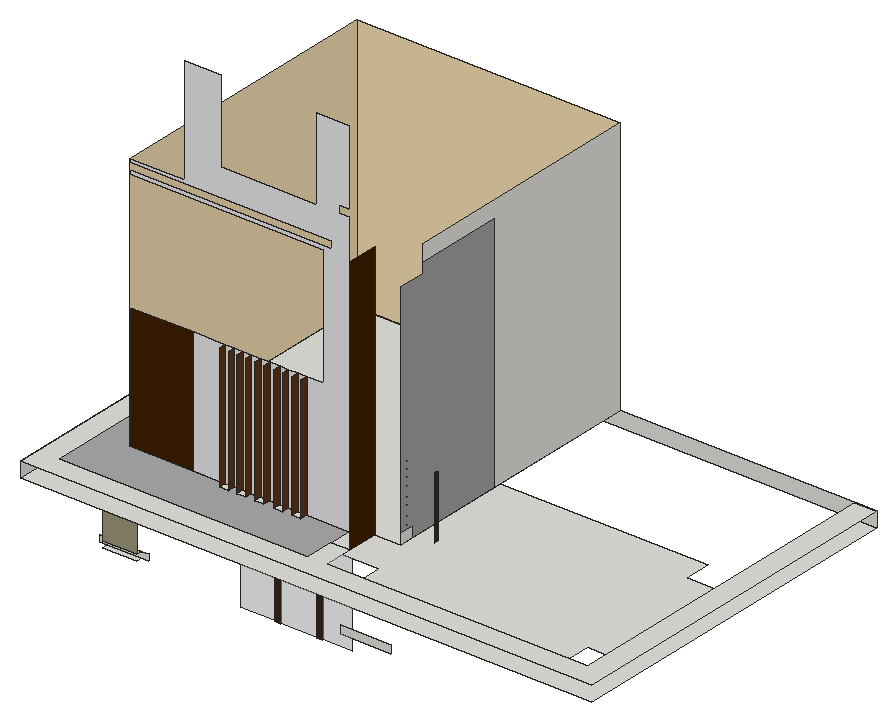
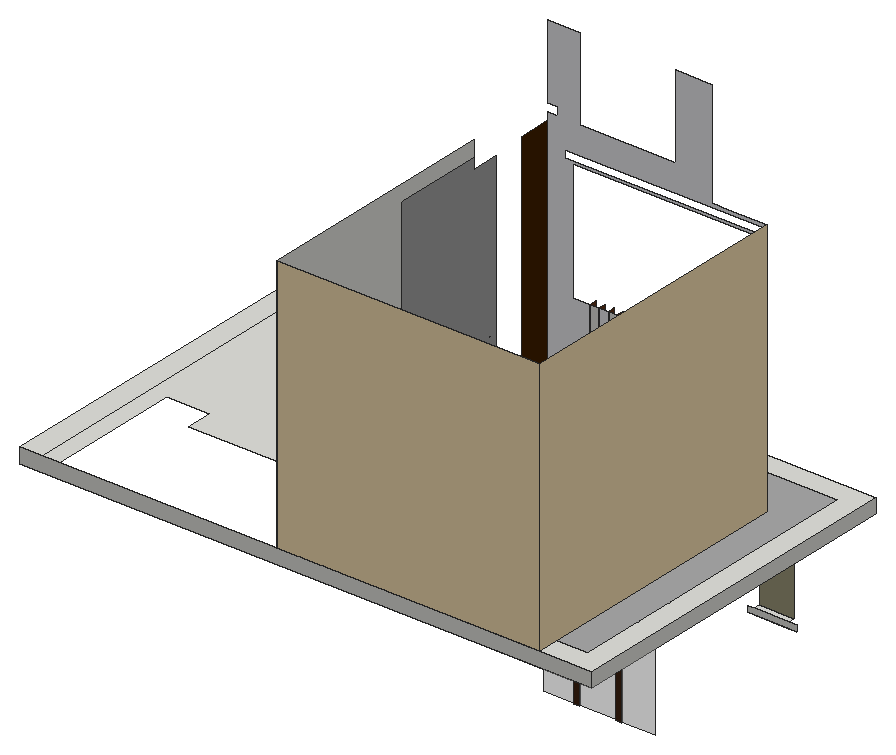
# SketchUp Ruby script. Lengths in inches.
U = 1.inch
M = Sketchup.active_model
def pt(a) = Geom::Point3d.new(a.map { |v| v * U })
def face(e, loops, mat)
  f = e.add_face(loops[0].map { |a| pt(a) })
  loops[1..].each { |l| e.add_face(l.map { |a| pt(a) }).erase! }
  f.material = f.back_material = mat if mat
  f
end
# faces: each face lists its corners as indices into pts; further lists are holes
def faces(e, pts, list, mat = nil) = list.each { |f| face(e, (f[0].is_a?(Array) ? f : [f]).map { |l| l.map { |i| pts[i] } }, mat) }
# xy, xz, yz: faces in a plane at the given z, y or x. An outline is a flat list of corners, or four numbers for a rectangle; further outlines are holes
def ring(l) = l.size == 4 ? [[l[0], l[1]], [l[2], l[1]], [l[2], l[3]], [l[0], l[3]]] : l.each_slice(2).to_a
def flat(e, list, mat, &to3) = list.each { |f| face(e, (f[0].is_a?(Array) ? f : [f]).map { |l| ring(l).map { |u, v| to3.(u, v) } }, mat) }
def xy(e, z, list, mat = nil) = flat(e, list, mat) { |x, y| [x, y, z] }
def xz(e, y, list, mat = nil) = flat(e, list, mat) { |x, z| [x, y, z] }
def yz(e, x, list, mat = nil) = flat(e, list, mat) { |y, z| [x, y, z] }
def lines(e, pts, list) = list.each { |a, b| e.add_line(pt(pts[a]), pt(pts[b])) }
# prism: a flat outline (further loops are holes) pulled along v
def prism(e, loops, v, mat = nil)
  f = face(e, loops, mat); d = Geom::Vector3d.new(v.map { |x| x * U })
  f.pushpull(f.normal.samedirection?(d) ? d.length : -d.length)
end
def box(e, o, s, mat = nil) = prism(e, [[o, [o[0] + s[0], o[1], o[2]], [o[0] + s[0], o[1] + s[1], o[2]], [o[0], o[1] + s[1], o[2]]]], [0, 0, s[2]], mat)
def at(x, y, z, deg = 0) = Geom::Transformation.translation(pt([x, y, z])) * Geom::Transformation.rotation(ORIGIN, Z_AXIS, deg.degrees)
def axes(o, x, y, z) = Geom::Transformation.new([*x, 0, *y, 0, *z, 0, *pt(o).to_a, 1])
def part(name) = M.definitions.add(name)
# library, detail: a bought-in or finely detailed component or shape, given as its bounding box
def library(name, o, s) = part(name).tap { |d| box(d.entities, o, s) }
def detail(e, o, s) = box(e.add_group.entities, o, s)
def put(e, d, t, mat = nil) = e.add_instance(d, t).tap { |i| i.material = mat if mat }
def group(e, t, mat = nil) = e.add_group.tap { |g| g.transformation = t; g.material = mat if mat }.entities
root = M.entities
M.materials.add("[0034_Wheat]").color = [245, 222, 179]
M.materials.add("[0136_Charcoal]").color = [35, 35, 35]
M.materials.add("[Blinds Vertical Pattern]").color = [232, 232, 234]
M.materials.add("[Blinds Vertical Stripe Gray]2").color = [160, 160, 160]
M.materials.add("[Color C08]").color = [63, 31, 0]
M.materials.add("[Color M03]").color = [170, 170, 170]
M.materials.add("[Stone Coursed Rough]").color = [155, 150, 122]
M.materials.add("[Translucent Glass Gray]").color = [178, 178, 178]
M.materials["[Translucent Glass Gray]"].alpha = 0.5
M.materials.add("[Wood Cherry Original]").color = [94, 53, 26]
M.materials.add("[Wood Veneer 01]").color = [63, 37, 19]
xy(root,93.02,[[55.77,217.98,71.76,220.79]])
xy(root,130.875,[[[41.9,187.36,41.9,352.92,55.77,352.92,55.77,263.99,164.37,263.99,164.37,292.92,277.86,292.92,277.86,280.61,297.85,280.61,297.85,352.92,308.53,352.92,308.53,187.36],[55.77,203.17,71.76,217.98],[281.86,203.17,297.85,217.98],[168.55,203.17,186.24,216.5]],[55.77,263.99,164.37,292.92],[55.77,292.92,164.37,292.92,164.37,343.79,64.9,343.79,64.9,352.92,55.77,352.92],[64.9,343.79,164.37,352.92]])
xy(root,137.875,[[41.9,187.36,308.53,187.36,308.53,352.92,298.6,352.92,298.6,197.29,176.75,197.29,176.75,210.73,168.19,210.73,168.19,197.29,51.83,197.29,51.83,342.99,66.16,342.99,66.16,352.92,41.9,352.92],[168.19,210.73,168.19,220.88,66.16,220.88,66.16,352.92,189.02,352.92,189.02,225.17,176.75,225.17,176.75,210.73],[110.6,217.51,114.76,220.88],[118.6,217.51,122.76,220.88],[127.16,217.51,131.32,220.88],
  [135.85,217.51,140.01,220.88],[144.35,217.51,148.51,220.88]])
xy(root,137.875,[[51.83,197.29,168.19,197.29,168.19,220.88,148.51,220.88,148.51,217.51,144.35,217.51,144.35,220.88,140.01,220.88,140.01,217.51,135.85,217.51,135.85,220.88,131.32,220.88,131.32,217.51,127.16,217.51,127.16,220.88,122.76,220.88,122.76,217.51,118.6,217.51,118.6,220.88,114.76,220.88,114.76,217.51,110.6,217.51,110.6,220.88,66.16,220.88,66.16,342.99,51.83,342.99]],"[Color M03]")
xz(root,217.98,[[55.77,95.8,55.77,130.875,71.76,130.875,71.76,95.87]],"[Stone Coursed Rough]")
xz(root,219.06,[[165.87,95.36,189.49,98.875]])
xz(root,220.79,[[52.21,93.02,52.21,95.8,55.77,95.8,71.76,95.87,74.94,95.87,74.94,93.02]])
xz(root,220.88,[[110.6,137.875,114.76,195.78],[118.6,137.875,122.76,195.78],[127.16,137.875,131.32,195.78],[135.85,137.875,140.01,195.78],[144.35,137.875,148.51,195.78]])
xz(root,220.88,[[148.51,137.875,168.19,137.875,168.19,269.25,163.51,269.25,163.51,272.9375,168.19,272.9375,168.19,307.625,153.36,307.625,153.36,269.1875,108.42,269.1875,108.42,307.625,91.59,307.625,91.59,258.0625,84.125,258.01,66.16,257.875,66.16,256.4,160.21,256.4,160.21,253.05,66.16,253.05,66.16,251.53,156.36,251.53,156.36,195.78,148.51,195.78],[95.83,137.875,110.6,195.78],[114.76,137.875,118.6,195.78],[122.76,137.875,127.16,195.78],[131.32,137.875,135.85,195.78],
  [140.01,137.875,144.35,195.78]],"[Blinds Vertical Pattern]")
xz(root,220.88,[[66.16,137.875,95.83,195.78]],"[Color C08]")
xz(root,263.99,[[83.47,57.46,99.06,113.58],[102.17,57.46,118.68,113.58],[121.79,57.46,135.84,113.58]],"[Translucent Glass Gray]")
xz(root,263.99,[[99.06,57.46,102.17,113.58],[118.68,57.46,121.79,113.58]],"[Wood Veneer 01]")
xz(root,352.92,[[41.9,130.875,308.53,137.875]])
xz(root,352.92,[[66.16,137.875,189.02,257.875]],"[0034_Wheat]")
yz(root,41.9,[[187.36,130.875,352.92,137.875]])
yz(root,66.16,[[220.88,137.875,352.92,257.875]],"[0034_Wheat]")
yz(root,110.6,[[217.51,137.875,220.88,195.78]],"[Wood Cherry Original]")
yz(root,114.76,[[217.51,137.875,220.88,195.78]],"[Wood Cherry Original]")
yz(root,118.6,[[217.51,137.875,220.88,195.78]],"[Wood Cherry Original]")
yz(root,122.76,[[217.51,137.875,220.88,195.78]],"[Wood Cherry Original]")
yz(root,127.16,[[217.51,137.875,220.88,195.78]],"[Wood Cherry Original]")
yz(root,131.32,[[217.51,137.875,220.88,195.78]],"[Wood Cherry Original]")
yz(root,135.85,[[217.51,137.875,220.88,195.78]],"[Wood Cherry Original]")
yz(root,140.01,[[217.51,137.875,220.88,195.78]],"[Wood Cherry Original]")
yz(root,144.35,[[217.51,137.875,220.88,195.78]],"[Wood Cherry Original]")
yz(root,148.51,[[217.51,137.875,220.88,195.78]],"[Wood Cherry Original]")
yz(root,176.75,[[210.73,137.875,225.17,257.875]],"[Color C08]")
yz(root,189.02,[[225.17,137.875,231.66,142.6875],[280.2,137.875,352.92,137.875,352.92,257.875,238.17,257.875,238.17,250.375,280.2,250.375]])
yz(root,189.02,[[[231.66,137.875,280.2,137.875,280.2,250.375,238.17,250.375,238.17,245.5,225.17,245.5,225.17,142.6875,231.66,142.6875],[228.53,170.81,228.36,170.83,228.21,170.89,228.08,170.99,227.98,171.12,227.92,171.27,227.9,171.43,227.92,171.59,227.98,171.74,228.08,171.875,228.21,171.97,228.36,172.04,228.53,172.06,228.6875,172.04,228.84,171.97,228.97,171.875,229.07,171.74,229.13,171.59,229.15,171.43,229.13,171.27,229.07,171.12,228.97,170.99,228.84,170.89,228.6875,170.83],[228.53,167.43,228.36,167.45,228.21,167.52,228.08,167.62,227.98,167.74,227.92,167.9,227.9,168.06,227.92,168.22,227.98,168.37,228.08,168.5,228.21,168.6,228.36,168.66,228.53,168.68,228.6875,168.66,228.84,168.6,228.97,168.5,229.07,168.37,229.13,168.22,229.15,168.06,229.13,167.9,229.07,167.74,228.97,167.62,228.84,167.52,228.6875,167.45],[228.53,163.93,228.36,163.95,228.21,164.02,228.08,164.12,227.98,164.24,227.92,164.4,227.9,164.56,227.92,164.72,227.98,164.87,228.08,165,228.21,165.1,228.36,165.16,228.53,165.18,228.6875,165.16,228.84,165.1,228.97,165,229.07,164.87,229.13,164.72,229.15,164.56,229.13,164.4,229.07,164.24,228.97,164.12,228.84,164.02,228.6875,163.95],[228.53,160.18,228.36,160.2,228.21,160.27,228.08,160.37,227.98,160.49,227.92,160.65,227.9,160.81,227.92,160.97,227.98,161.12,228.08,161.25,228.21,161.35,228.36,161.41,228.53,161.43,228.6875,161.41,228.84,161.35,228.97,161.25,229.07,161.12,229.13,160.97,229.15,160.81,229.13,160.65,229.07,160.49,228.97,160.37,228.84,160.27,228.6875,160.2],[228.53,155.62,228.36,155.64,228.21,155.7,228.08,155.8,227.98,155.93,227.92,156.08,227.9,156.24,227.92,156.41,227.98,156.56,228.08,156.6875,228.21,156.79,228.36,156.85,228.53,156.87,228.6875,156.85,228.84,156.79,228.97,156.6875,229.07,156.56,229.13,156.41,229.15,156.24,229.13,156.08,229.07,155.93,228.97,155.8,228.84,155.7,228.6875,155.64],[228.53,152.12,228.36,152.14,228.21,152.2,228.08,152.3,227.98,152.43,227.92,152.58,227.9,152.74,227.92,152.91,227.98,153.06,228.08,153.1875,228.21,153.29,228.36,153.35,228.53,153.37,228.6875,153.35,228.84,153.29,228.97,153.1875,229.07,153.06,229.13,152.91,229.15,152.74,229.13,152.58,229.07,152.43,228.97,152.3,228.84,152.2,228.6875,152.14],[228.53,143.87,228.36,143.89,228.21,143.95,228.08,144.05,227.98,144.18,227.92,144.33,227.9,144.49,227.92,144.66,227.98,144.81,228.08,144.9375,228.21,145.04,228.36,145.1,228.53,145.12,228.6875,145.1,228.84,145.04,228.97,144.9375,229.07,144.81,229.13,144.66,229.15,144.49,229.13,144.33,229.07,144.18,228.97,144.05,228.84,143.95,228.6875,143.89],[228.53,147.74,228.36,147.77,228.21,147.83,228.08,147.93,227.98,148.06,227.92,148.21,227.9,148.37,227.92,148.53,227.98,148.68,228.08,148.8125,228.21,148.91,228.36,148.97,228.53,148.99,228.6875,148.97,228.84,148.91,228.97,148.8125,229.07,148.68,229.13,148.53,229.15,148.37,229.13,148.21,229.07,148.06,228.97,147.93,228.84,147.83,228.6875,147.77],[228.44,174.54,228.3,174.5625,228.16,174.62,228.04,174.71,227.95,174.83,227.9,174.96,227.88,175.11,227.9,175.25,227.95,175.39,228.04,175.5,228.16,175.59,228.3,175.65,228.44,175.67,228.59,175.65,228.72,175.59,228.84,175.5,228.93,175.39,228.98,175.25,229,175.11,228.98,174.96,228.93,174.83,228.84,174.71,228.72,174.62,228.59,174.5625]]],"[Blinds Vertical Stripe Gray]2")
p = [[55.77,217.98,95.8],[71.76,217.98,95.87],[71.76,220.79,95.87],[55.77,220.79,95.8],[202.86,227.76,142.6875],[203.05,227.61,142.6875],
  [203.05,227.61,171.43],[202.86,227.76,171.43],[202.71,227.96,142.6875],[202.75,227.9,171.43],[202.71,227.96,171.43],[202.61,228.18,142.6875],
  [202.61,228.18,171.43],[202.58,228.42,142.6875],[202.58,228.42,171.43],[202.61,228.67,142.6875],[202.61,228.67,171.43],[202.71,228.89,142.6875],
  [202.71,228.89,171.43],[202.86,229.09,142.6875],[202.86,229.09,171.43],[203.05,229.24,142.6875],[202.94,229.15,171.43],[203.05,229.24,171.43]]
faces(root,p,[[0,1,2,3]])
faces(root,p,[[4,5,6,7],[8,4,7,9,10],[11,8,10,12],[13,11,12,14],[15,13,14,16],[17,15,16,18],[19,17,18,20],[21,19,20,22,23]],"[0136_Charcoal]")
